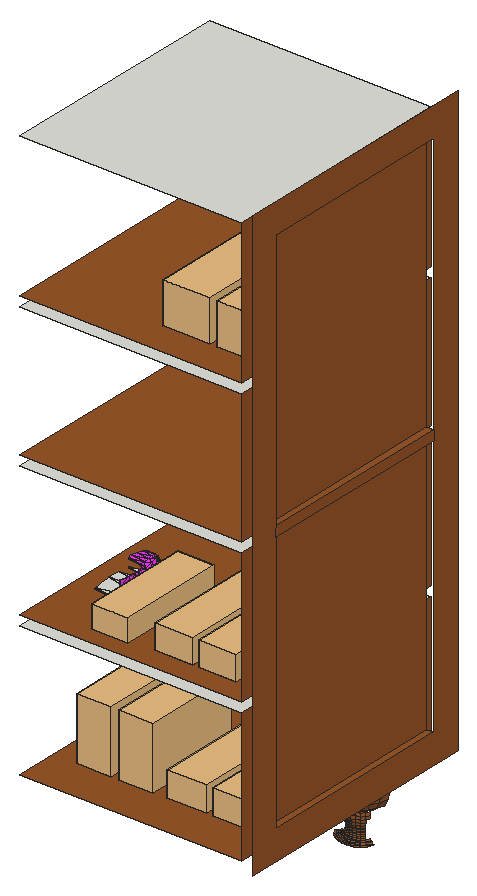
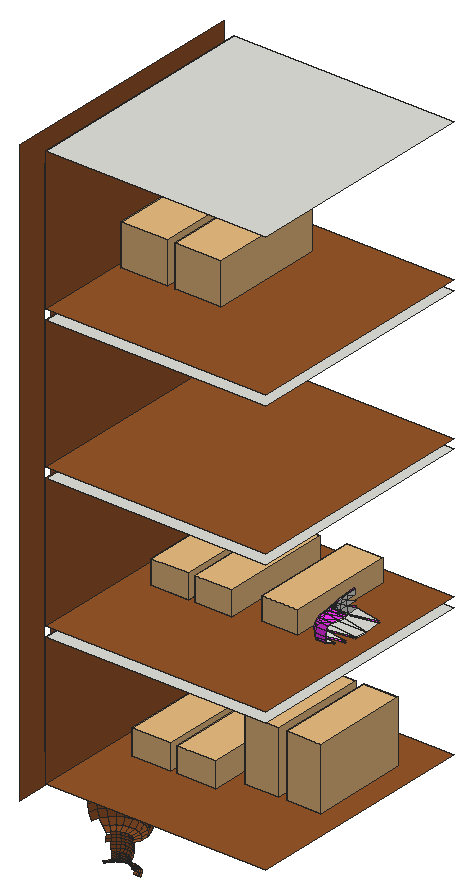
# SketchUp Ruby script. Lengths in inches.
U = 1.inch
M = Sketchup.active_model
def pt(a) = Geom::Point3d.new(a.map { |v| v * U })
def face(e, loops, mat)
  f = e.add_face(loops[0].map { |a| pt(a) })
  loops[1..].each { |l| e.add_face(l.map { |a| pt(a) }).erase! }
  f.material = f.back_material = mat if mat
  f
end
# faces: each face lists its corners as indices into pts; further lists are holes
def faces(e, pts, list, mat = nil) = list.each { |f| face(e, (f[0].is_a?(Array) ? f : [f]).map { |l| l.map { |i| pts[i] } }, mat) }
# xy, xz, yz: faces in a plane at the given z, y or x. An outline is a flat list of corners, or four numbers for a rectangle; further outlines are holes
def ring(l) = l.size == 4 ? [[l[0], l[1]], [l[2], l[1]], [l[2], l[3]], [l[0], l[3]]] : l.each_slice(2).to_a
def flat(e, list, mat, &to3) = list.each { |f| face(e, (f[0].is_a?(Array) ? f : [f]).map { |l| ring(l).map { |u, v| to3.(u, v) } }, mat) }
def xy(e, z, list, mat = nil) = flat(e, list, mat) { |x, y| [x, y, z] }
def xz(e, y, list, mat = nil) = flat(e, list, mat) { |x, z| [x, y, z] }
def yz(e, x, list, mat = nil) = flat(e, list, mat) { |y, z| [x, y, z] }
def lines(e, pts, list) = list.each { |a, b| e.add_line(pt(pts[a]), pt(pts[b])) }
# prism: a flat outline (further loops are holes) pulled along v
def prism(e, loops, v, mat = nil)
  f = face(e, loops, mat); d = Geom::Vector3d.new(v.map { |x| x * U })
  f.pushpull(f.normal.samedirection?(d) ? d.length : -d.length)
end
def box(e, o, s, mat = nil) = prism(e, [[o, [o[0] + s[0], o[1], o[2]], [o[0] + s[0], o[1] + s[1], o[2]], [o[0], o[1] + s[1], o[2]]]], [0, 0, s[2]], mat)
def at(x, y, z, deg = 0) = Geom::Transformation.translation(pt([x, y, z])) * Geom::Transformation.rotation(ORIGIN, Z_AXIS, deg.degrees)
def axes(o, x, y, z) = Geom::Transformation.new([*x, 0, *y, 0, *z, 0, *pt(o).to_a, 1])
def part(name) = M.definitions.add(name)
# library, detail: a bought-in or finely detailed component or shape, given as its bounding box
def library(name, o, s) = part(name).tap { |d| box(d.entities, o, s) }
def detail(e, o, s) = box(e.add_group.entities, o, s)
def put(e, d, t, mat = nil) = e.add_instance(d, t).tap { |i| i.material = mat if mat }
def group(e, t, mat = nil) = e.add_group.tap { |g| g.transformation = t; g.material = mat if mat }.entities
root = M.entities
M.materials.add("[Color A03]").color = [255, 101, 101]
M.materials.add("[Color G05]").color = [0, 255, 0]
M.materials.add("[Color I03]").color = [101, 101, 255]
M.materials.add("[Color K04]").color = [255, 50, 255]
M.materials.add("[Wood Cherry Original]").color = [152, 86, 42]
c1 = library("Group\#4",[0,0,0],[9.05,3.05,1.93])
c2 = library("Group\#71",[0,0,0],[9.05,3.05,1.93])
c3 = library("Group\#49",[0,0,0],[9.05,3.05,1.93])
c4 = library("Group\#6",[0,0,0],[16.85,6.02,10.8125])
c5 = library("Group\#8",[0,0,0],[16.85,6.02,10.8125])
c6 = library("Group\#19",[0,0,0],[5.49,13.47,5.24])
c7 = library("skpCFE",[-1.94,0.63,-0.92],[9.04,3.05,1.94])
c8 = library("Group\#1",[0,0,0],[73.99,73.99,3])
c9 = part("Group\#43")
p = [[51.915,68.666,0.026],[51.894,68.676,0.026],[3.278,51.855,0.026],[0,38.173,0.026],[3.287,51.865,0.026],[68.666,20.052,0.026],
  [68.676,20.073,0.026],[51.914,68.635,0],[51.914,68.648,0.011],[51.913,68.661,1.207],[51.876,68.638,1.207],[59.709,34.52,10.914],
  [59.717,34.52,10.91],[59.714,34.527,10.91],[51.917,68.668,0.026],[51.913,68.661,0.026],[68.668,20.051,0.026],[51.936,68.655,0.026],
  [68.655,20.031,0.026],[59.722,34.526,10.905]]
lines(c9.entities,p,[[0,1],[2,3],[4,2],[5,6],[7,8],[9,10],[11,12],[13,12],[8,0],[14,1],[1,15],[5,16],
  [16,6],[17,0],[18,5],[17,14],[18,16],[13,19]])
detail(c9.entities,[0,0,0],[71.97,71.97,12.3])
xy(root,14.078,[[179.354,46.115,201.807,70.115]],"[Wood Cherry Original]")
xy(root,16.078,[[202.151,49.115,202.901,69.115]],"[Wood Cherry Original]")
xy(root,27.578,[[179.354,46.115,201.807,70.115]])
xy(root,28.578,[[181.341,53.115,184.07,53.661,184.234,54.424,184.446,55.117,184.522,55.924,181.135,56.291,181.063,55.195,181.165,54.137]])
xy(root,28.578,[[[179.354,46.115,201.807,70.115],[181.341,53.115,181.165,54.137,181.063,55.195,181.135,56.291,184.522,55.924,184.446,55.117,184.234,54.424,184.07,53.661]]],"[Wood Cherry Original]")
xy(root,42.078,[[179.354,46.115,201.807,70.115]])
xy(root,42.578,[[202.151,49.115,202.901,69.115]],"[Wood Cherry Original]")
xy(root,43.078,[[179.354,46.115,201.807,70.115]],"[Wood Cherry Original]")
xy(root,43.578,[[202.151,49.115,202.901,69.115]],"[Wood Cherry Original]")
xy(root,56.578,[[179.354,46.115,201.807,70.115]])
xy(root,57.578,[[179.354,46.115,201.807,70.115]],"[Wood Cherry Original]")
xy(root,70.078,[[202.151,49.115,202.901,69.115]])
xy(root,72.078,[[179.354,46.115,201.807,70.115]])
yz(root,201.807,[[46.115,14.078,70.115,27.578],[46.115,28.578,70.115,42.078],[46.115,43.078,70.115,56.578],[46.115,57.578,70.115,72.078]],"[Wood Cherry Original]")
yz(root,202.151,[[49.115,16.078,69.115,42.578],[49.115,43.578,69.115,70.078]],"[Wood Cherry Original]")
yz(root,202.901,[[[46.115,13.078,72.115,73.078],[49.115,16.078,69.115,70.078]],[49.115,42.578,69.115,43.578]],"[Wood Cherry Original]")
p = [[196.698,64.879,6.002],[196.639,64.739,6],[197.178,64.593,6],[197.199,64.743,6.002],[197.737,64.59,6],[197.717,64.741,6.002],
  [198.276,64.733,6],[198.219,64.873,6.002],[196.25,65.14,6.002],[196.157,65.02,6],[196.755,65.016,6.029],[197.219,64.89,6.029],
  [197.699,64.888,6.029],[198.163,65.011,6.029],[198.761,65.01,6],[198.669,65.131,6.002],[196.341,65.258,6.029],[196.81,65.147,6.082],
  [197.238,65.031,6.082],[197.681,65.029,6.082],[198.109,65.142,6.082],[198.579,65.249,6.029],[195.884,65.508,6.002],[195.764,65.417,6],
  [196.427,65.37,6.082],[198.493,65.362,6.082],[199.158,65.403,6],[199.038,65.496,6.002],[196.003,65.598,6.029],[198.92,65.587,6.029],
  [198.808,65.674,6.082],[196.115,65.684,6.082],[195.626,65.959,6.002],[195.486,65.901,6],[199.439,65.886,6],[199.299,65.944,6.002],
  [195.764,66.015,6.029],[199.162,66.002,6.029],[195.895,66.069,6.082],[199.031,66.057,6.082],[196.861,65.268,6.158],[197.255,65.16,6.158],
  [197.664,65.159,6.158],[198.059,65.263,6.158],[196.507,65.473,6.158],[198.414,65.466,6.158],[196.219,65.764,6.158],[198.704,65.754,6.158],
  [196.016,66.118,6.158],[198.91,66.107,6.158],[196.905,65.374,6.255],[197.271,65.275,6.255],[197.649,65.273,6.255],[198.016,65.37,6.255],
  [196.578,65.565,6.255],[198.344,65.558,6.255],[196.311,65.833,6.255],[198.613,65.825,6.255],[198.804,66.152,6.255],[196.943,65.463,6.37],
  [197.284,65.37,6.37],[197.637,65.369,6.37],[197.979,65.459,6.37],[196.637,65.641,6.37],[198.286,65.635,6.37],[196.388,65.892,6.37],
  [198.537,65.884,6.37],[196.972,65.532,6.501],[197.294,65.445,6.501],[197.628,65.444,6.501],[197.95,65.529,6.501],[196.683,65.701,6.501],
  [198.24,65.694,6.501],[196.448,65.9375,6.501],[198.477,65.93,6.501],[196.991,65.58,6.642],[197.301,65.496,6.642],[197.621,65.494,6.642],
  [197.931,65.576,6.642],[196.714,65.741,6.642],[198.209,65.735,6.642],[196.489,65.969,6.642],[198.437,65.961,6.642],[197.001,65.604,6.79],
  [197.304,65.521,6.79],[197.618,65.52,6.79],[197.921,65.6,6.79],[196.73,65.762,6.79],[198.193,65.756,6.79],[196.509,65.984,6.79],
  [198.416,65.977,6.79],[197.001,65.603,6.94],[197.304,65.521,6.94],[197.618,65.52,6.94],[197.921,65.6,6.94],[196.73,65.761,6.94],
  [198.194,65.756,6.94],[196.509,65.984,6.94],[198.416,65.977,6.94],[196.991,65.579,7.088],[197.301,65.495,7.088],[197.621,65.494,7.088],
  [197.931,65.575,7.088],[196.714,65.74,7.088],[198.21,65.735,7.088],[196.488,65.968,7.088],[198.437,65.961,7.088],[196.971,65.531,7.229],
  [197.294,65.443,7.229],[197.628,65.442,7.229],[197.951,65.527,7.229],[196.682,65.699,7.229],[198.241,65.693,7.229],[196.447,65.937,7.229],
  [198.478,65.929,7.229],[196.928,65.429,7.509],[197.279,65.333,7.509],[197.642,65.332,7.509],[197.993,65.425,7.509],[196.614,65.611,7.509],
  [198.308,65.605,7.509],[196.358,65.869,7.509],[198.566,65.861,7.509],[196.899,65.359,7.801],[197.268,65.258,7.801],[197.651,65.256,7.801],
  [198.022,65.354,7.801],[196.568,65.551,7.801],[198.354,65.544,7.801],[198.626,65.814,7.801],[196.298,65.823,7.801],[196.883,65.322,8.099],
  [197.263,65.219,8.099],[197.657,65.217,8.099],[198.037,65.317,8.099],[196.543,65.52,8.099],[198.378,65.513,8.099],[196.266,65.799,8.099],
  [198.658,65.79,8.099],[196.882,65.319,8.4],[197.263,65.216,8.4],[197.657,65.214,8.4],[198.038,65.315,8.4],[196.542,65.518,8.4],
  [198.38,65.511,8.4],[196.264,65.797,8.4],[198.66,65.788,8.4],[196.068,66.14,8.4],[196.071,66.141,8.099],[198.856,66.13,8.099],
  [198.858,66.129,8.4],[196.895,65.351,8.699],[197.267,65.249,8.699],[197.653,65.248,8.699],[198.025,65.346,8.699],[196.5625,65.545,8.699],
  [198.36,65.538,8.699],[196.291,65.818,8.699],[198.633,65.809,8.699],[198.827,66.142,8.699],[196.923,65.416,8.992],[197.277,65.319,8.992],
  [197.644,65.318,8.992],[197.998,65.411,8.992],[198.317,65.594,8.992],[196.606,65.6,8.992],[196.347,65.861,8.992],[198.577,65.852,8.992],
  [196.651,64.768,9.209],[197.182,64.623,9.209],[197.733,64.621,9.209],[198.265,64.762,9.209],[196.176,65.045,9.209],[198.742,65.035,9.209],
  [195.788,65.435,9.209],[199.133,65.422,9.209],[195.515,65.913,9.209],[196.165,66.179,8.992],[198.762,66.169,8.992],[199.41,65.898,9.209],
  [196.428,64.234,9.659],[197.105,64.05,9.659],[197.806,64.047,9.659],[198.484,64.226,9.659],[195.822,64.587,9.659],[199.093,64.574,9.659],
  [195.328,65.085,9.659],[199.591,65.068,9.659],[194.979,65.694,9.659],[199.944,65.674,9.659],[196.281,63.883,10.284],[197.053,63.673,10.284],
  [197.854,63.67,10.284],[198.628,63.874,10.284],[195.589,64.286,10.284],[199.323,64.271,10.284],[195.025,64.854,10.284],[199.892,64.835,10.284],
  [200.295,65.527,10.284],[194.627,65.549,10.284],[200.128,66.351,9.659],[200.505,66.3,10.284],[197.06,53.261,11.001],[197.077,53.13,10.284],
  [196.303,52.925,10.284],[196.252,53.048,11.001],[198.702,53.039,11.001],[198.65,52.916,10.284],[197.878,53.127,10.284],[197.895,53.258,11.001],
  [196.23,63.761,11.001],[197.036,63.541,11.001],[197.871,63.538,11.001],[198.679,63.751,11.001],[195.508,64.181,11.001],[199.404,64.166,11.001],
  [194.919,64.774,11.001],[199.997,64.754,11.001],[194.505,65.499,11.001],[200.417,65.476,11.001],[194.291,66.307,11.001],[194.423,66.324,10.284],
  [200.636,66.282,11.001],[197.077,53.13,11.719],[196.303,52.925,11.719],[198.65,52.916,11.719],[197.878,53.127,11.719],[196.281,63.883,11.719],
  [197.053,63.673,11.719],[197.854,63.67,11.719],[198.628,63.874,11.719],[195.589,64.286,11.719],[199.323,64.271,11.719],[195.025,64.854,11.719],
  [199.892,64.835,11.719],[194.627,65.549,11.719],[200.295,65.527,11.719],[194.423,66.324,11.719],[200.505,66.3,11.719],[196.428,64.234,12.343],
  [197.105,64.05,12.343],[197.806,64.047,12.343],[198.484,64.226,12.343],[195.822,64.587,12.343],[199.093,64.574,12.343],[195.328,65.085,12.343],
  [199.591,65.068,12.343],[199.944,65.674,12.343],[194.979,65.694,12.343],[200.128,66.351,12.343],[196.651,64.768,12.793],[197.182,64.623,12.793],
  [197.733,64.621,12.793],[198.265,64.762,12.793],[196.176,65.045,12.793],[198.742,65.035,12.793],[195.788,65.435,12.793],[199.133,65.422,12.793],
  [195.515,65.913,12.793],[199.41,65.898,12.793],[196.923,65.416,13.01],[197.277,65.319,13.01],[197.644,65.318,13.01],[197.998,65.411,13.01],
  [196.606,65.6,13.01],[198.317,65.594,13.01],[196.347,65.861,13.01],[198.577,65.852,13.01],[196.165,66.179,13.01],[198.762,66.169,13.01],
  [197.206,66.093,12.967],[197.375,66.047,12.967],[197.551,66.046,12.967],[197.72,66.091,12.967],[197.055,66.181,12.967],[197.872,66.178,12.967],
  [184.896,56.888,15.482],[184.857,56.893,15.465],[184.778,56.988,15.622],[186.279,56.888,15.482],[186.397,56.988,15.622],[186.319,56.893,15.465],
  [188.988,55.649,16.547],[188.946,55.619,16.551],[188.948,55.647,16.536],[187.303,57,16.617],[187.513,56.968,16.682],[187.497,56.948,16.687],
  [187.292,56.885,16.666],[183.924,56.642,16.765],[183.679,56.948,16.687],[183.641,56.959,16.691],[183.64,56.698,16.806],[183.641,56.965,16.688],
  [183.662,56.968,16.682],[187.534,56.995,16.675],[187.535,56.965,16.688],[188.9375,55.192,16.782],[188.909,55.159,16.791],[188.911,55.191,16.776],
  [183.939,56.372,16.909],[183.668,56.416,16.943],[183.671,56.388,16.959],[183.701,56.359,16.971],[183.948,56.117,17.069],[187.474,56.359,16.971],
  [187.504,56.388,16.959],[187.508,56.416,16.943],[187.236,56.372,16.909],[187.227,56.117,17.069],[187.258,56.391,16.894],[187.514,56.461,16.914],
  [184.634,54.601,17.037],[184.603,54.596,17.031],[184.601,54.619,17.021],[186.542,54.601,17.037],[186.574,54.619,17.021],[186.572,54.596,17.031],
  [188.549,55.95,17.209],[188.598,56.229,16.991],[188.554,55.951,17.202],[188.553,55.951,17.203],[188.045,56.239,17.093],[187.819,56.378,16.994],
  [187.837,56.391,16.987],[188.056,56.345,17.028],[183.4,56.404,16.975],[183.357,56.378,16.994],[183.339,56.391,16.987],[183.676,56.355,16.979],
  [188.71,55.217,17.364],[188.706,55.292,17.358],[188.713,55.267,17.336],[188.706,55.303,17.357],[188.715,55.291,17.323],[184.378,55.098,17.429],
  [184.385,55.007,17.483],[184.372,55.019,17.519],[186.797,55.098,17.429],[186.804,55.019,17.519],[186.79,55.007,17.483],[184.811,53.876,18.5625],
  [184.811,53.876,18.574],[184.826,53.804,18.594],[184.834,53.834,17.622],[186.341,53.834,17.622],[186.349,53.804,18.594],[186.364,53.876,18.574],
  [186.364,53.876,18.5625],[184.891,53.433,18.333],[184.873,53.069,18.4375],[184.874,53.074,18.475],[184.889,53.346,18.609],[186.286,53.346,18.609],
  [186.302,53.074,18.475],[186.303,53.069,18.4375],[186.285,53.433,18.333],[189.054,53.433,18.333],[189,53.069,18.4375],[189.001,53.074,18.475],
  [189.042,53.346,18.609],[184.784,53.975,18.692],[184.795,53.93,18.688],[184.784,53.935,18.688],[184.771,53.983,18.693],[184.773,53.984,18.693],
  [186.402,53.984,18.693],[186.404,53.983,18.693],[186.392,53.935,18.688],[186.381,53.93,18.688],[186.392,53.975,18.692],[188.986,53.986,18.693],
  [189.005,53.968,18.692],[189.01,53.931,18.688],[188.995,53.929,18.688],[184.779,53.899,19.075],[184.758,53.989,19.016],[184.755,54.007,18.991],
  [184.804,53.802,19.06],[184.791,53.846,19.11],[186.371,53.802,19.06],[186.421,54.007,18.991],[186.417,53.989,19.016],[186.396,53.899,19.075],
  [186.384,53.846,19.11],[181.341,53.115,28.578],[184.07,53.661,28.578],[184.101,52.64,28.66],[184.153,53.678,28.658],[184.18,52.653,28.74],
  [184.234,54.424,28.578],[184.319,54.432,28.658],[184.446,55.117,28.578],[184.528,55.115,28.658],[184.522,55.924,28.578],[184.603,55.916,28.658],
  [184.381,56.88,28.579],[181.135,56.291,28.578],[184.467,56.867,28.658],[184.005,57.948,28.62],[181.349,57.354,28.616],[184.11,57.936,28.698],
  [181.793,58.205,28.679],[182.48,58.615,28.722],[183.361,58.579,28.722],[184.048,52.64,28.791],[184.019,53.67,28.71],[181.392,53.129,28.709],
  [184.174,53.701,29.363],[184.18,52.653,28.956],[184.153,53.678,28.873],[184.277,54.469,29.353],[184.183,54.437,28.709],[184.319,54.432,28.873],
  [184.39,55.128,28.707],[181.12,55.196,28.708],[184.403,55.151,29.337],[184.528,55.115,28.873],[184.465,55.922,28.707],[181.191,56.281,28.708],
  [184.478,55.933,29.334],[184.603,55.916,28.873],[184.326,56.863,28.708],[184.344,56.865,29.332],[184.467,56.867,28.873],[181.403,57.329,28.745],
  [183.958,57.902,28.745],[184.001,57.902,29.33],[184.11,57.936,28.913],[182.495,58.543,28.843],[181.835,58.149,28.802],[183.337,58.507,28.842],
  [183.345,58.575,29.329],[183.396,58.657,28.813],[183.396,58.657,29.029],[182.459,58.695,28.813],[182.489,58.607,29.328],[182.459,58.695,29.029],
  [184.313,53.691,29.338],[184.416,54.447,29.338],[184.543,55.129,29.338],[184.619,55.9375,29.338],[184.481,56.898,29.338],[184.121,57.978,29.338],
  [183.4,58.705,29.338],[182.454,58.744,29.338],[184.288,52.661,29.381],[184.358,53.698,29.893],[184.431,54.429,29.855],[184.498,55.087,29.855],
  [184.363,55.1,29.812],[184.441,55.869,29.802],[184.572,55.873,29.855],[184.313,56.778,29.794],[184.403,56.912,29.855],[183.978,57.79,29.792],
  [184.088,57.856,29.855],[183.336,58.45,29.786],[183.388,58.563,29.855],[182.5,58.481,29.785],[182.468,58.6,29.855],[184.217,53.704,29.893],
  [184.148,52.653,29.401],[184.29,54.438,29.839],[184.196,54.401,30.304],[184.135,55.075,30.19],[184.185,55.851,30.123],[184.073,56.716,30.037],
  [183.758,57.655,30.058],[183.226,58.194,30.041],[182.567,58.217,30.042],[184.19,53.708,30.386],[184.193,52.698,29.964],[184.335,52.699,29.968],
  [184.328,53.707,30.457],[184.323,54.404,30.389],[184.225,55.074,30.315],[184.266,55.866,30.239],[184.063,56.969,30.188],[183.822,57.692,30.179],
  [183.256,58.264,30.161],[182.549,58.292,30.161],[184.134,52.744,30.471],[184.267,52.744,30.554],[183.686,56.482,30.14],[183.604,56.82,30.099],
  [183.34,57.731,30.141],[182.506,57.831,30.159],[184.052,55.708,30.18],[183.586,56.085,30.21],[182.243,56.261,30.209],[182.161,56.634,30.173],
  [182.241,57.075,30.139],[184.157,55.073,30.274],[184.025,55.668,30.257],[184.049,55.679,30.333],[183.584,56.095,30.278],[183.595,56.107,30.357],
  [183.704,56.502,30.348],[182.253,56.2,30.277],[183.589,57.086,30.31],[183.411,57.74,30.264],[182.381,57.864,30.282],[184.244,54.4,30.375],
  [182.246,56.207,30.357],[182.149,56.645,30.352],[182.245,57.259,30.327],[184.248,53.708,30.451],[184.188,52.747,30.541]]
faces(root,p,[[0,1,2,3],[3,2,4,5],[5,4,6,7],[8,9,1,0],[10,0,3,11],[11,3,5,12],[12,5,7,13],[7,6,14,15],
  [16,8,0,10],[17,10,11,18],[18,11,12,19],[19,12,13,20],[13,7,15,21],[22,23,9,8],[24,16,10,17],[20,13,21,25],
  [15,14,26,27],[28,22,8,16],[21,15,27,29],[25,21,29,30],[31,28,16,24],[32,33,23,22],[27,26,34,35],[36,32,22,28],
  [29,27,35,37],[38,36,28,31],[30,29,37,39],[40,17,18,41],[41,18,19,42],[42,19,20,43],[44,24,17,40],[43,20,25,45],
  [46,31,24,44],[45,25,30,47],[48,38,31,46],[47,30,39,49],[50,40,41,51],[51,41,42,52],[52,42,43,53],[54,44,40,50],
  [53,43,45,55],[56,46,44,54],[55,45,47,57],[57,47,49,58],[59,50,51,60],[60,51,52,61],[61,52,53,62],[63,54,50,59],
  [62,53,55,64],[65,56,54,63],[64,55,57,66],[67,59,60,68],[68,60,61,69],[69,61,62,70],[71,63,59,67],[70,62,64,72],
  [73,65,63,71],[72,64,66,74],[75,67,68,76],[76,68,69,77],[77,69,70,78],[79,71,67,75],[78,70,72,80],[81,73,71,79],
  [80,72,74,82],[83,75,76,84],[84,76,77,85],[85,77,78,86],[87,79,75,83],[86,78,80,88],[89,81,79,87],[88,80,82,90],
  [91,83,84,92],[92,84,85,93],[93,85,86,94],[95,87,83,91],[94,86,88,96],[97,89,87,95],[96,88,90,98],[99,91,92,100],
  [100,92,93,101],[101,93,94,102],[103,95,91,99],[102,94,96,104],[105,97,95,103],[104,96,98,106],[107,99,100,108],[108,100,101,109],
  [109,101,102,110],[111,103,99,107],[110,102,104,112],[113,105,103,111],[112,104,106,114],[115,107,108,116],[116,108,109,117],[117,109,110,118],
  [119,111,107,115],[118,110,112,120],[121,113,111,119],[120,112,114,122],[123,115,116,124],[124,116,117,125],[125,117,118,126],[127,119,115,123],
  [126,118,120,128],[128,120,122,129],[130,121,119,127],[131,123,124,132],[132,124,125,133],[133,125,126,134],[135,127,123,131],[134,126,128,136],
  [137,130,127,135],[136,128,129,138],[139,131,132,140],[140,132,133,141],[141,133,134,142],[143,135,131,139],[142,134,136,144],[145,137,135,143],
  [144,136,138,146],[147,148,137,145],[146,138,149,150],[151,139,140,152],[152,140,141,153],[153,141,142,154],[155,143,139,151],[154,142,144,156],
  [157,145,143,155],[156,144,146,158],[158,146,150,159],[160,151,152,161],[161,152,153,162],[162,153,154,163],[163,154,156,164],[165,155,151,160],
  [166,157,155,165],[164,156,158,167],[168,160,161,169],[169,161,162,170],[170,162,163,171],[172,165,160,168],[171,163,164,173],[174,166,165,172],
  [173,164,167,175],[176,177,166,174],[175,167,178,179],[180,168,169,181],[181,169,170,182],[182,170,171,183],[184,172,168,180],[183,171,173,185],
  [186,174,172,184],[185,173,175,187],[188,176,174,186],[187,175,179,189],[190,180,181,191],[191,181,182,192],[192,182,183,193],[194,184,180,190],
  [193,183,185,195],[196,186,184,194],[195,185,187,197],[197,187,189,198],[199,188,186,196],[198,189,200,201],[202,203,204,205],[206,207,208,209],
  [209,208,203,202],[210,190,191,211],[211,191,192,212],[212,192,193,213],[214,194,190,210],[213,193,195,215],[216,196,194,214],[215,195,197,217],
  [218,199,196,216],[217,197,198,219],[220,221,199,218],[219,198,201,222],[223,202,205,224],[225,206,209,226],[226,209,202,223],[227,210,211,228],
  [228,211,212,229],[229,212,213,230],[231,214,210,227],[230,213,215,232],[233,216,214,231],[232,215,217,234],[235,218,216,233],[234,217,219,236],
  [237,220,218,235],[236,219,222,238],[239,227,228,240],[240,228,229,241],[241,229,230,242],[243,231,227,239],[242,230,232,244],[245,233,231,243],
  [244,232,234,246],[246,234,236,247],[248,235,233,245],[247,236,238,249],[250,239,240,251],[251,240,241,252],[252,241,242,253],[254,243,239,250],
  [253,242,244,255],[256,245,243,254],[255,244,246,257],[258,248,245,256],[257,246,247,259],[260,250,251,261],[261,251,252,262],[262,252,253,263],
  [264,254,250,260],[263,253,255,265],[266,256,254,264],[265,255,257,267],[268,258,256,266],[267,257,259,269],[270,260,261,271],[271,261,262,272],
  [272,262,263,273],[274,264,260,270],[273,263,265,275]],"[Wood Cherry Original]")
faces(root,p,[[276,277,278],[279,280,281],[282,283,284],[285,286,287,288],[289,290,291,292],[290,291,293,294],[293,291,290,294],[295,286,296],
  [297,298,299],[300,301,302,303,304],[305,306,307,308,309],[307,306,305,310,311],[312,313,314],[315,316,317],[318,319,320,321],[322,323,324,325],
  [326,327,328],[329,302,303],[330,331,332],[332,331,333,334],[334,332,331,333],[335,336,337],[338,339,340],[341,342,343,344],
  [345,346,347,348],[349,350,351,352],[353,354,355,356],[357,358,359,360],[361,362,363,364,365],[364,365,361,362,363],[366,367,368,369,370],[370,366,367,368,369],
  [371,372,373,374],[375,376,377,378,379],[380,381,382,383,384],[405,406,407],[408,406,405],[406,408,411],[411,412,406],[412,414,415],
  [412,411,416],[416,414,412],[415,414,418,419],[414,416,420],[420,418,414],[419,418,422],[418,420,423],[423,422,418],
  [425,422,426],[422,423,427],[427,426,422],[429,430,426],[426,431,429],[426,427,432],[432,431,426],[436,429,431],
  [431,432,436],[450,416,411],[416,450,451],[451,420,416],[420,451,453],[453,423,420],[423,453,455],[455,427,423],
  [427,455,457],[457,432,427],[432,457,459],[459,436,432],[461,408,462],[408,461,463],[463,411,408],[411,463,450],
  [464,463,461],[463,464,465],[465,450,463],[450,465,466],[466,451,450],[451,466,467],[467,453,451],[453,467,468],
  [468,455,453],[455,468,469],[469,457,455],[469,470,459,457],[471,461,472],[461,471,464],[472,482,471],[467,466,484],
  [484,485,467],[468,467,485],[469,486,487],[486,469,468],[487,470,469],[488,466,465],[466,488,489],[466,489,484],
  [489,490,484],[490,491,484],[485,484,491],[491,492,485],[486,485,492],[485,486,468],[492,487,486],[493,465,464],
  [465,493,494],[494,488,465],[488,494,496],[496,489,488],[499,490,489],[489,496,499],[503,464,471],[464,503,493],
  [493,503,475],[475,476,493],[494,493,476],[476,495,494],[496,494,495],[495,497,496],[497,504,499],[499,496,497],
  [507,471,482],[503,507,474],[471,507,503],[474,475,503],[482,508,507],[507,508,483],[483,474,507]])
faces(root,p,[[385,386,387],[386,388,389],[388,386,390],[390,391,388],[391,390,392],[392,393,391],[392,394,395,393],[396,394,397],
  [395,394,396],[396,398,395],[399,396,400],[398,396,399],[399,401,398],[399,402,403],[403,404,399],[401,399,404],
  [409,389,388,410],[410,388,391,413],[413,391,393,417],[417,393,395,421],[421,395,398,424],[424,398,401,428],[428,401,433,434],[404,433,401],
  [433,404,403],[403,435,433],[434,433,435,437],[409,410,438],[439,438,410],[410,413,439],[440,439,413],[413,417,440],
  [440,417,421,441],[441,421,424,442],[443,442,424],[424,428,443],[444,443,428],[428,434,444],[444,434,437,445],[446,438,447],
  [448,447,438],[438,439,448],[449,448,439],[439,440,449],[449,440,441,452],[454,452,441],[441,442,454],[454,442,443,456],
  [456,443,444,458],[458,444,445,460],[473,447,474],[475,474,447],[447,448,475],[476,475,448],[448,449,476],[477,476,449],
  [449,452,477],[478,477,452],[452,454,478],[479,478,454],[454,456,479],[480,479,456],[456,458,480],[480,458,460,481],
  [474,483,473],[476,477,495],[497,495,477],[477,498,497],[498,477,478],[478,500,498],[500,478,479],[479,501,500],
  [502,501,480],[479,480,501],[480,481,502],[504,497,498],[498,505,504],[505,498,500],[500,506,505],[506,500,501],
  [501,502,506]],"[Color K04]")
put(root,c1,axes([188.87,47.89,28.58],[0,1.2,0],[-1.2,0,0],[0,0,1.2]),"[Color K04]")
put(root,c2,axes([191.2,48.375,28.58],[0,1.25,0],[1.25,0,0],[0,0,1.25]),"[Color G05]")
put(root,c3,axes([199.4375,48.375,28.58],[0,1.25,0],[-1.25,0,0],[0,0,1.25]),"[Color G05]")
put(root,c4,axes([181.7,60.16,14.08],[0,-0.58378,0],[0.58378,0,0],[0,0,0.58378]),"[Color A03]")
put(root,c5,axes([185.97,60.16,14.08],[0,-0.58378,0],[0.58378,0,0],[0,0,0.58378]),"[Color A03]")
put(root,c6,axes([191.17,61.08,57.21],[0.86175,0,0],[0,-0.86175,0],[0,0,0.86175]),"[Wood Cherry Original]")
put(root,c6,axes([201.38,61.08,57.21],[-0.86175,0,0],[0,-0.86175,0],[0,0,0.86175]),"[Wood Cherry Original]")
put(root,c7,axes([195.58,52.98,15.27],[0,1.3,0],[-1.3,0,0],[0,0,1.3]),"[Color I03]")
put(root,c7,axes([194.59,52.98,15.27],[0,1.3,0],[1.3,0,0],[0,0,1.3]),"[Color I03]")
put(root,c8,axes([188.06,56.15,30.37],[-0.00023,0.02884,-0.00243],[-0.02891,-0.00012,0.00131],[0.00129,0.00244,0.02881]))
put(root,c9,axes([194.1875,57.07,30.33],[0,0.02509,0],[-0.03153,0,0],[0,0,0.03153]))
put(root,c9,axes([198.67,57.07,30.33],[0,0.02509,0],[-0.03153,0,0],[0,0,0.03153]))
